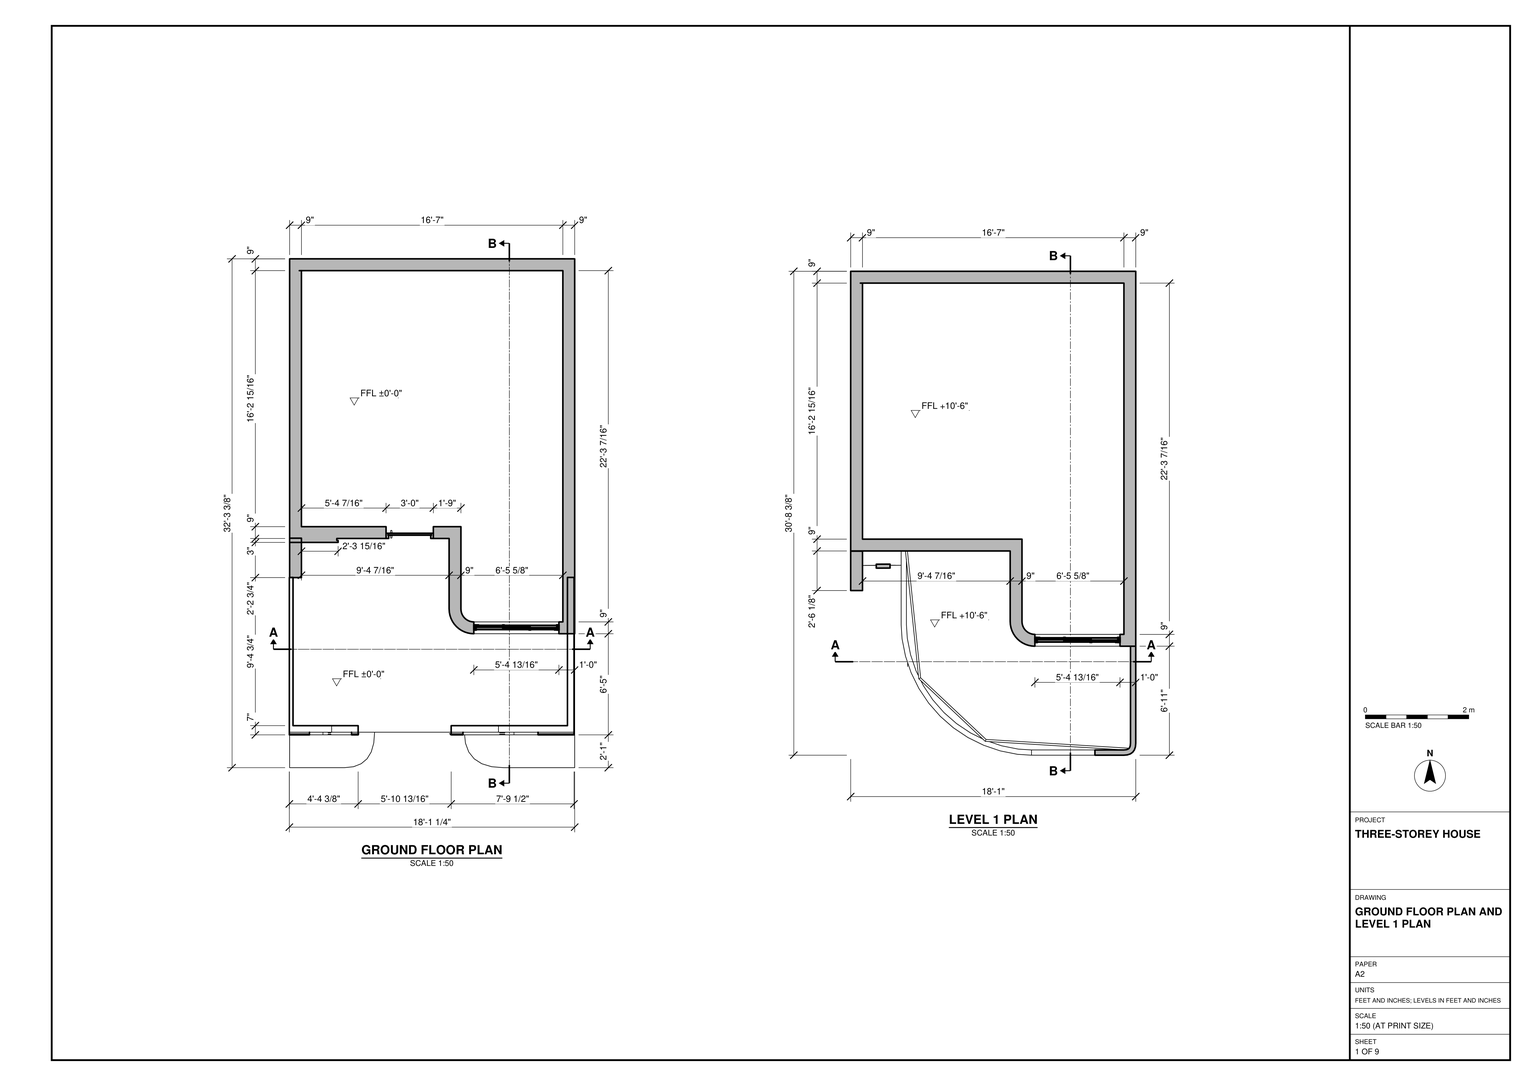
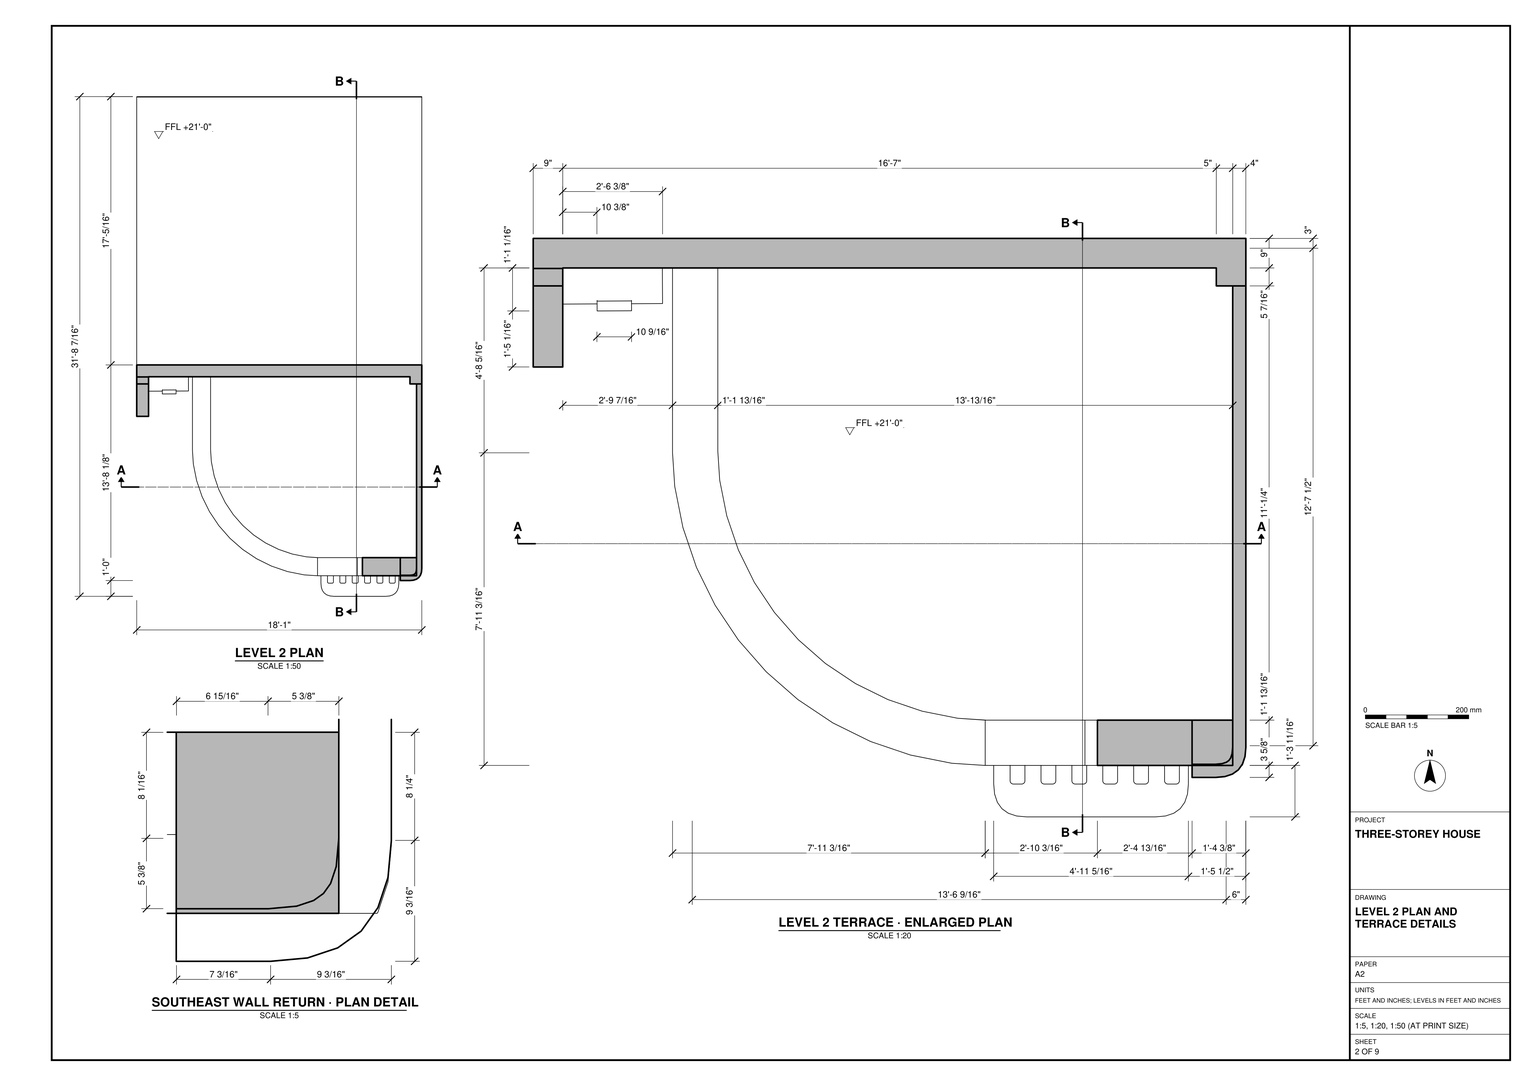
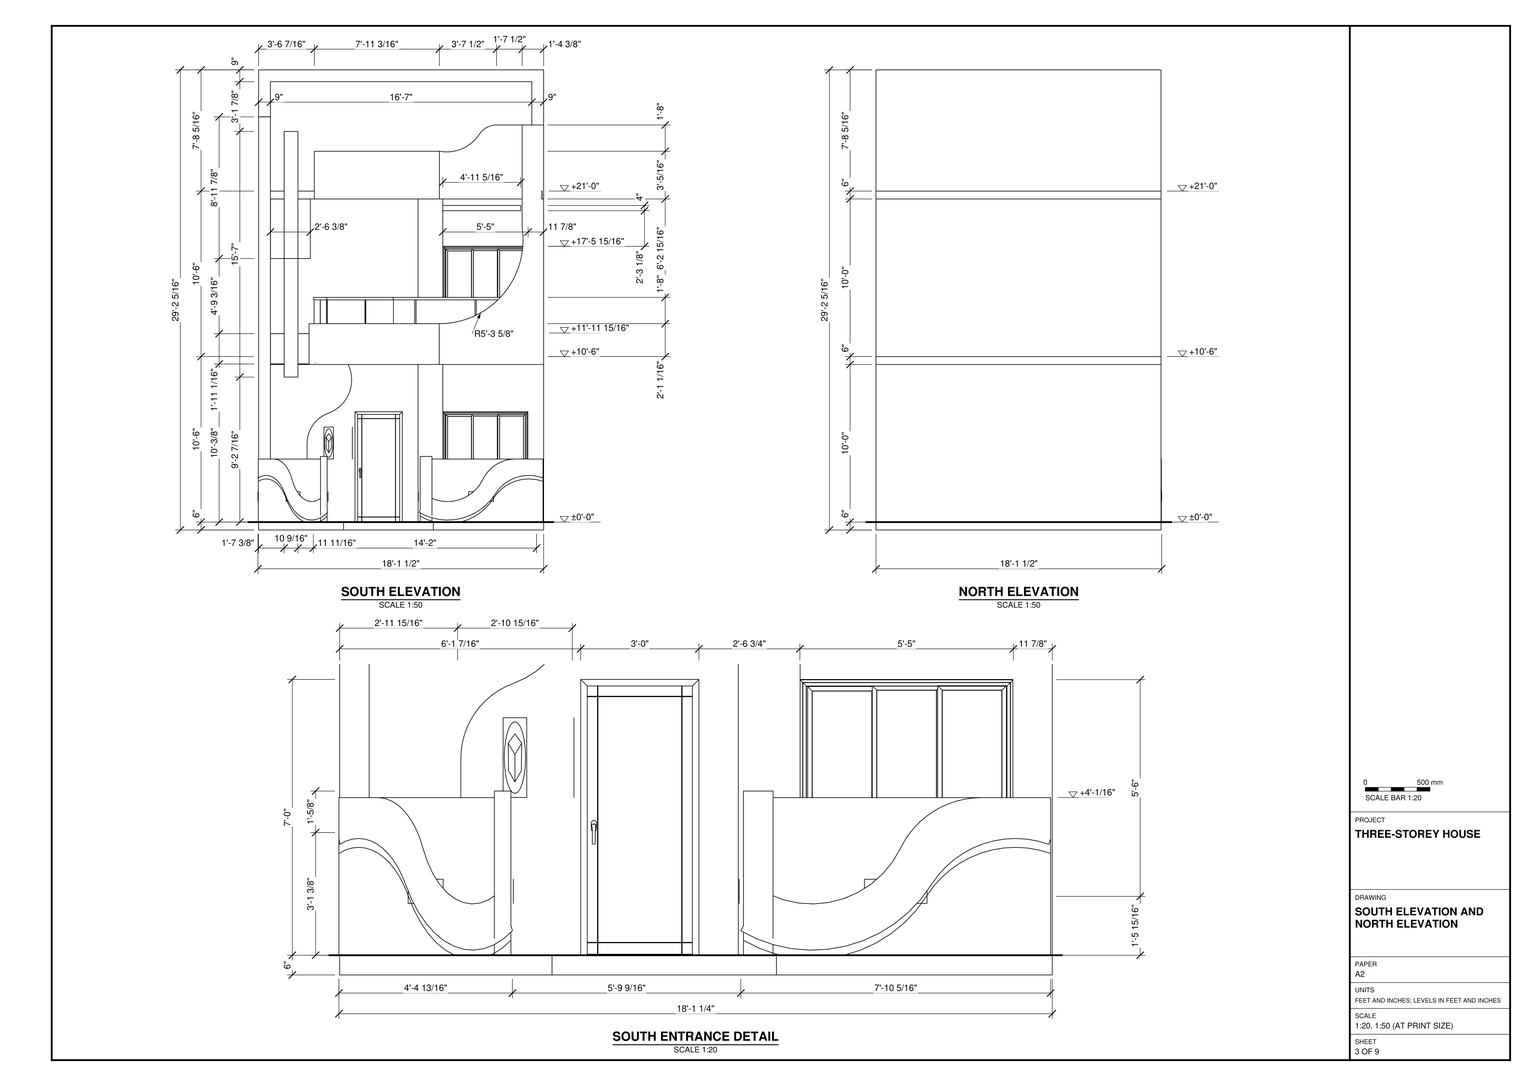
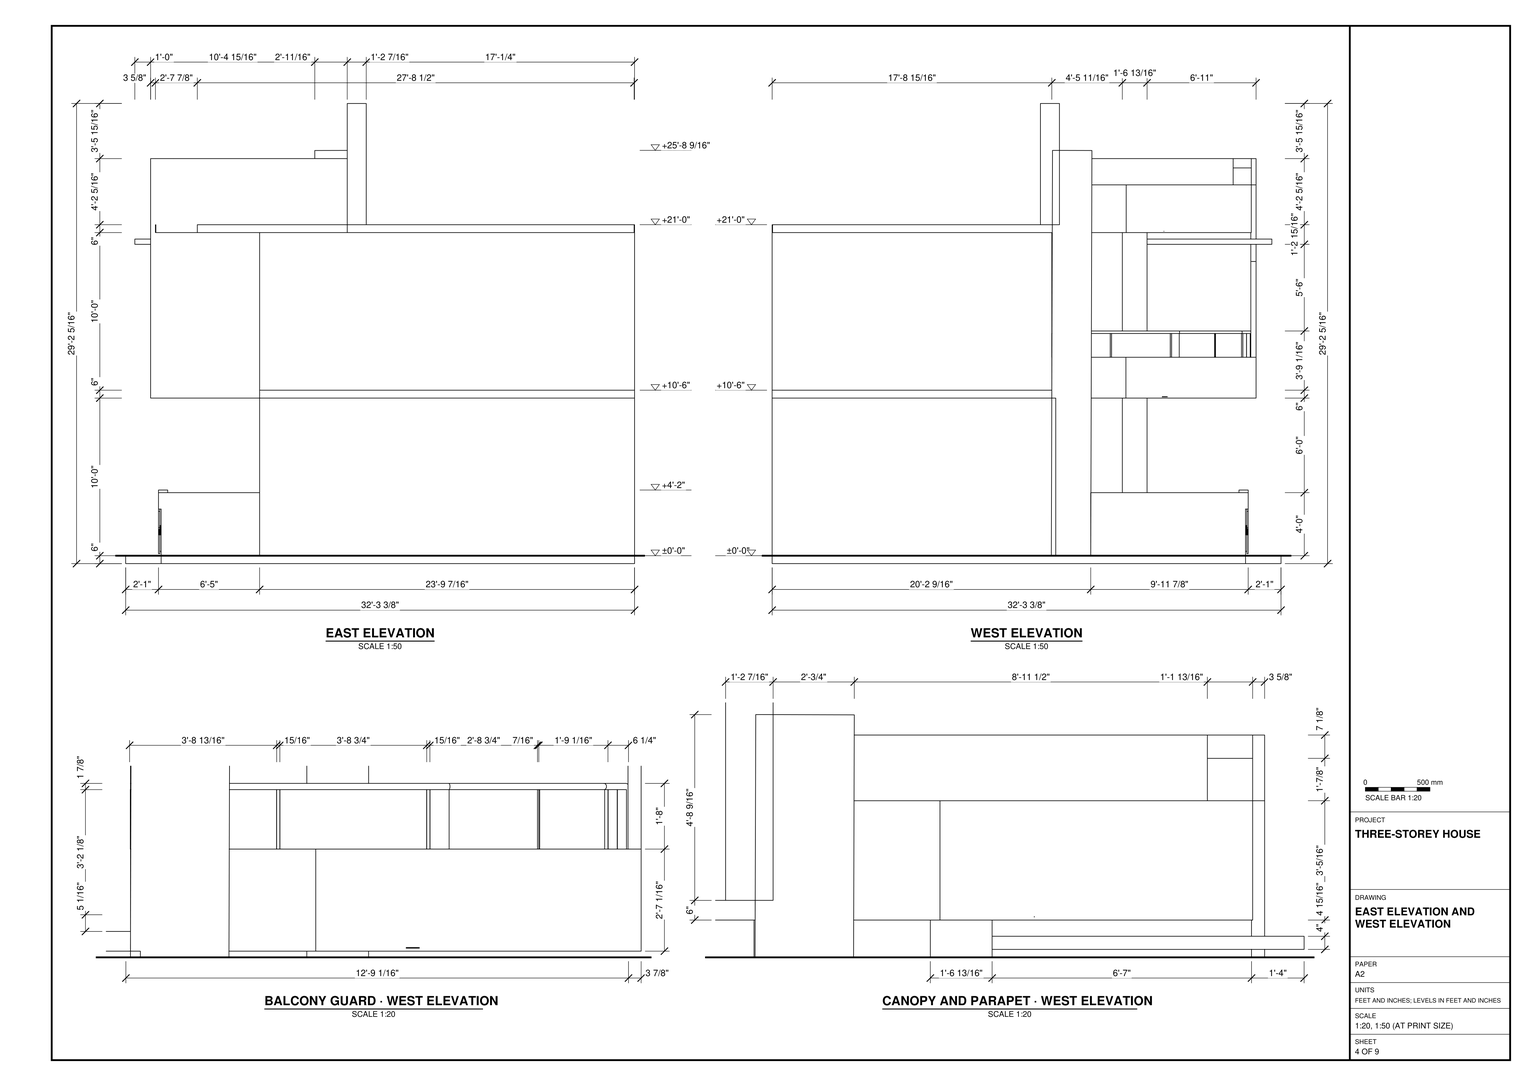
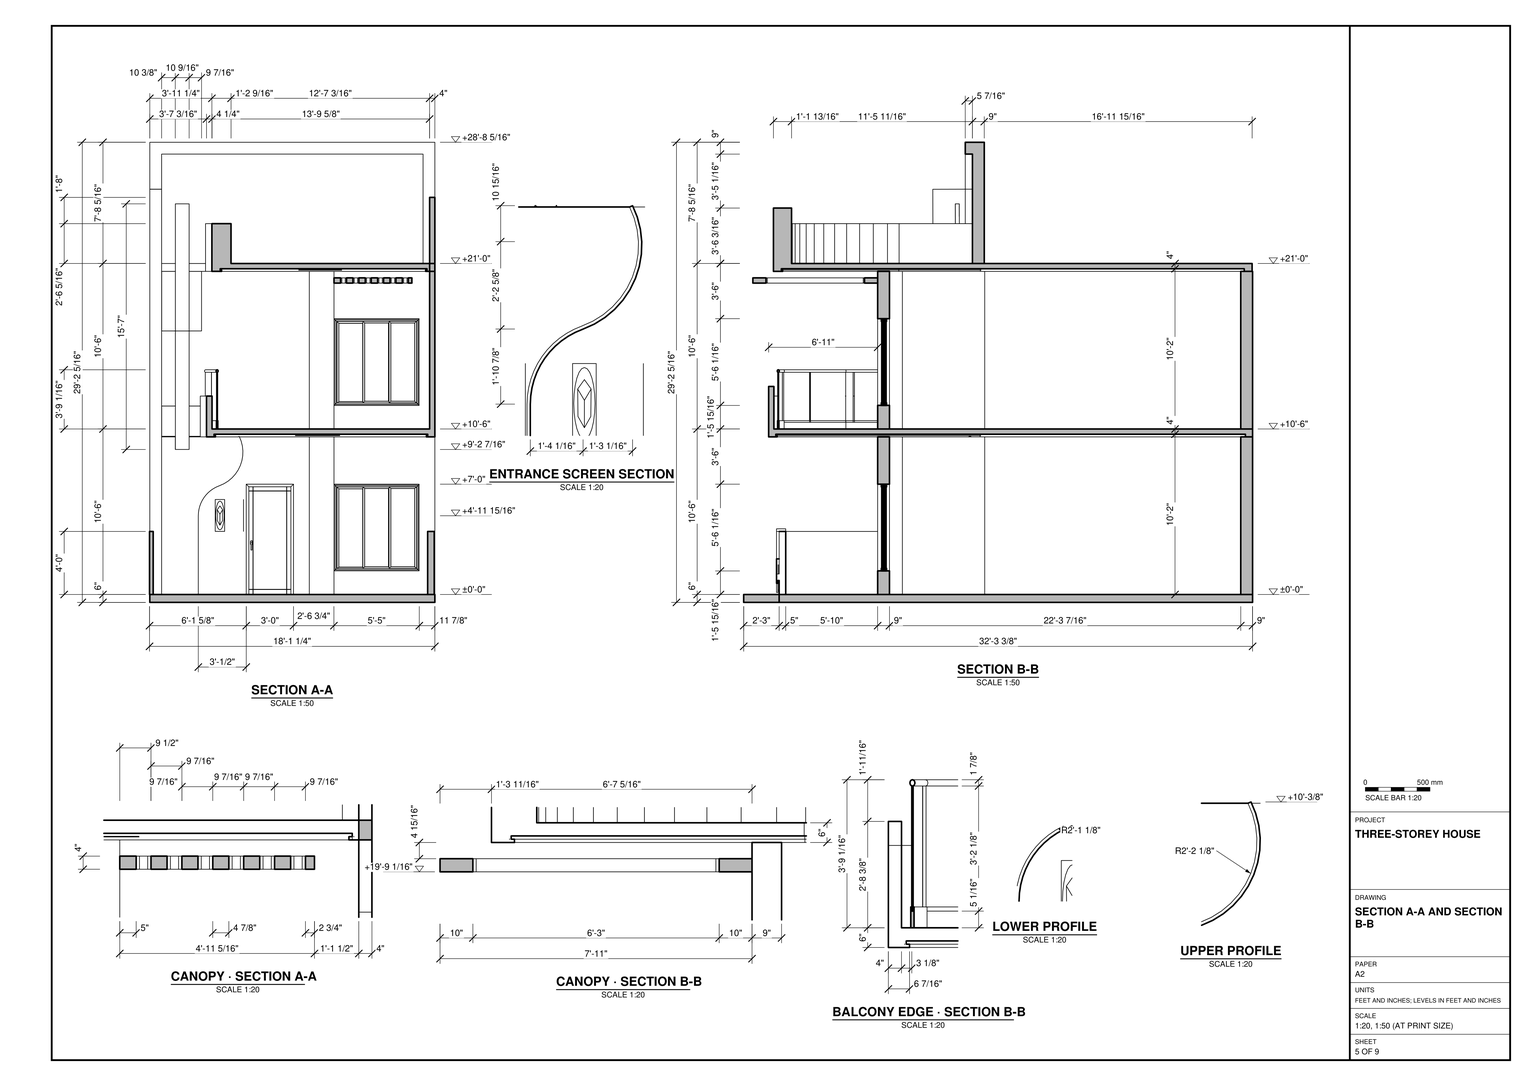
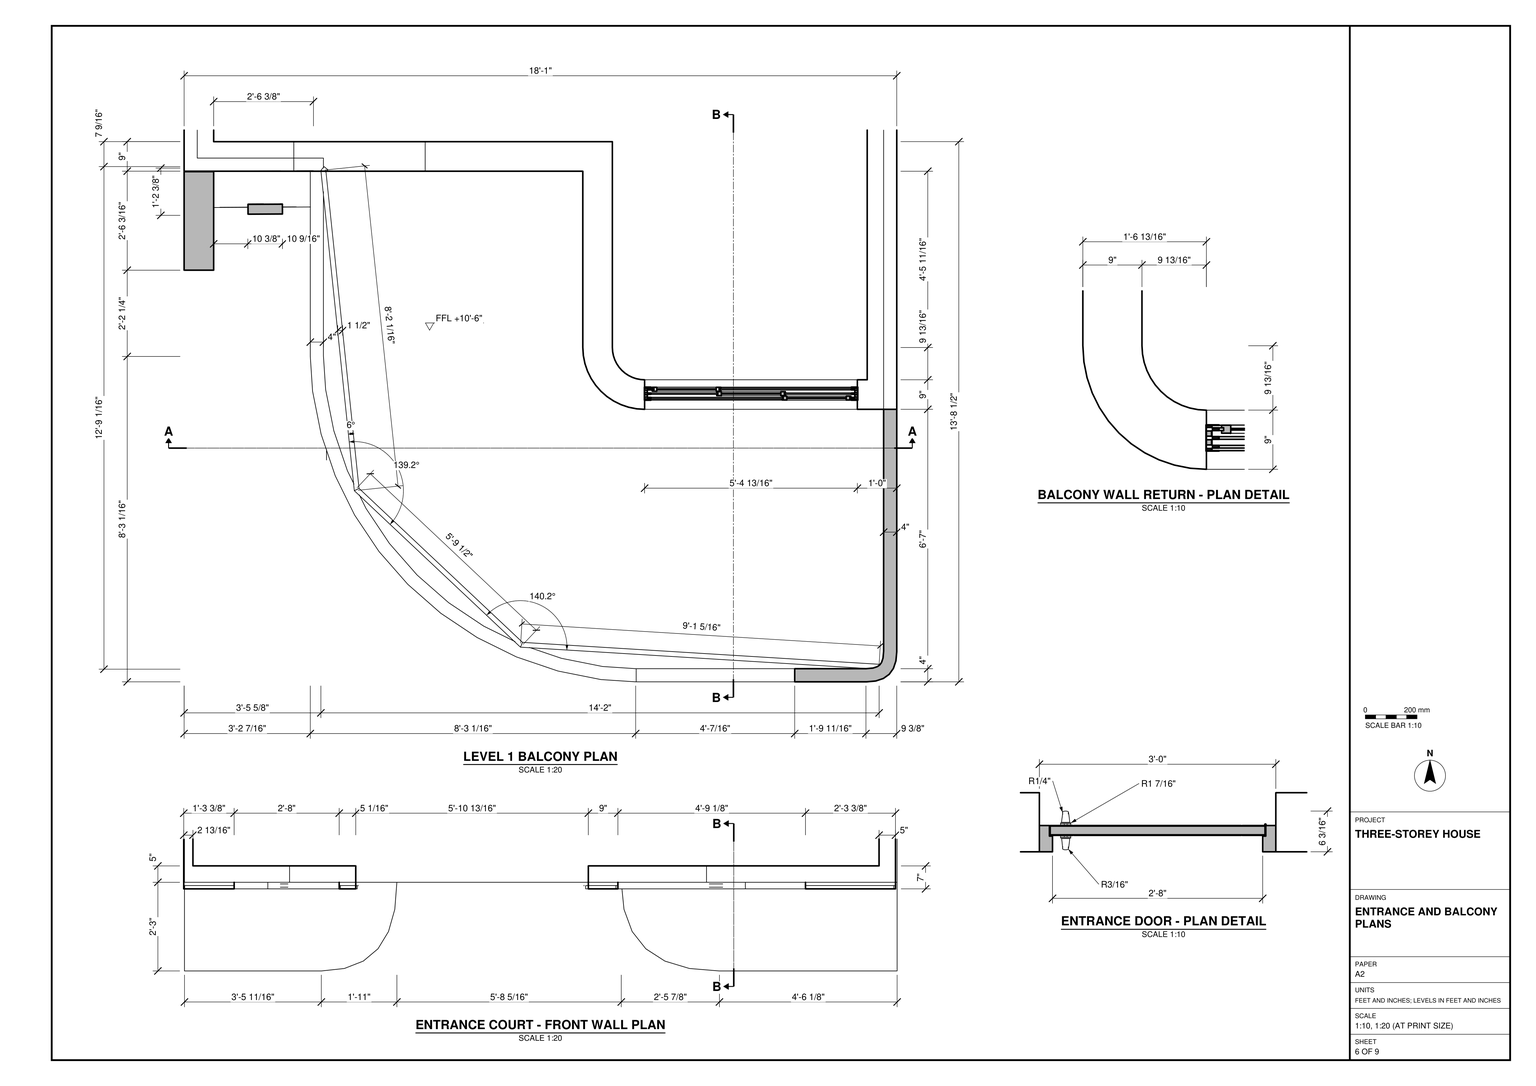
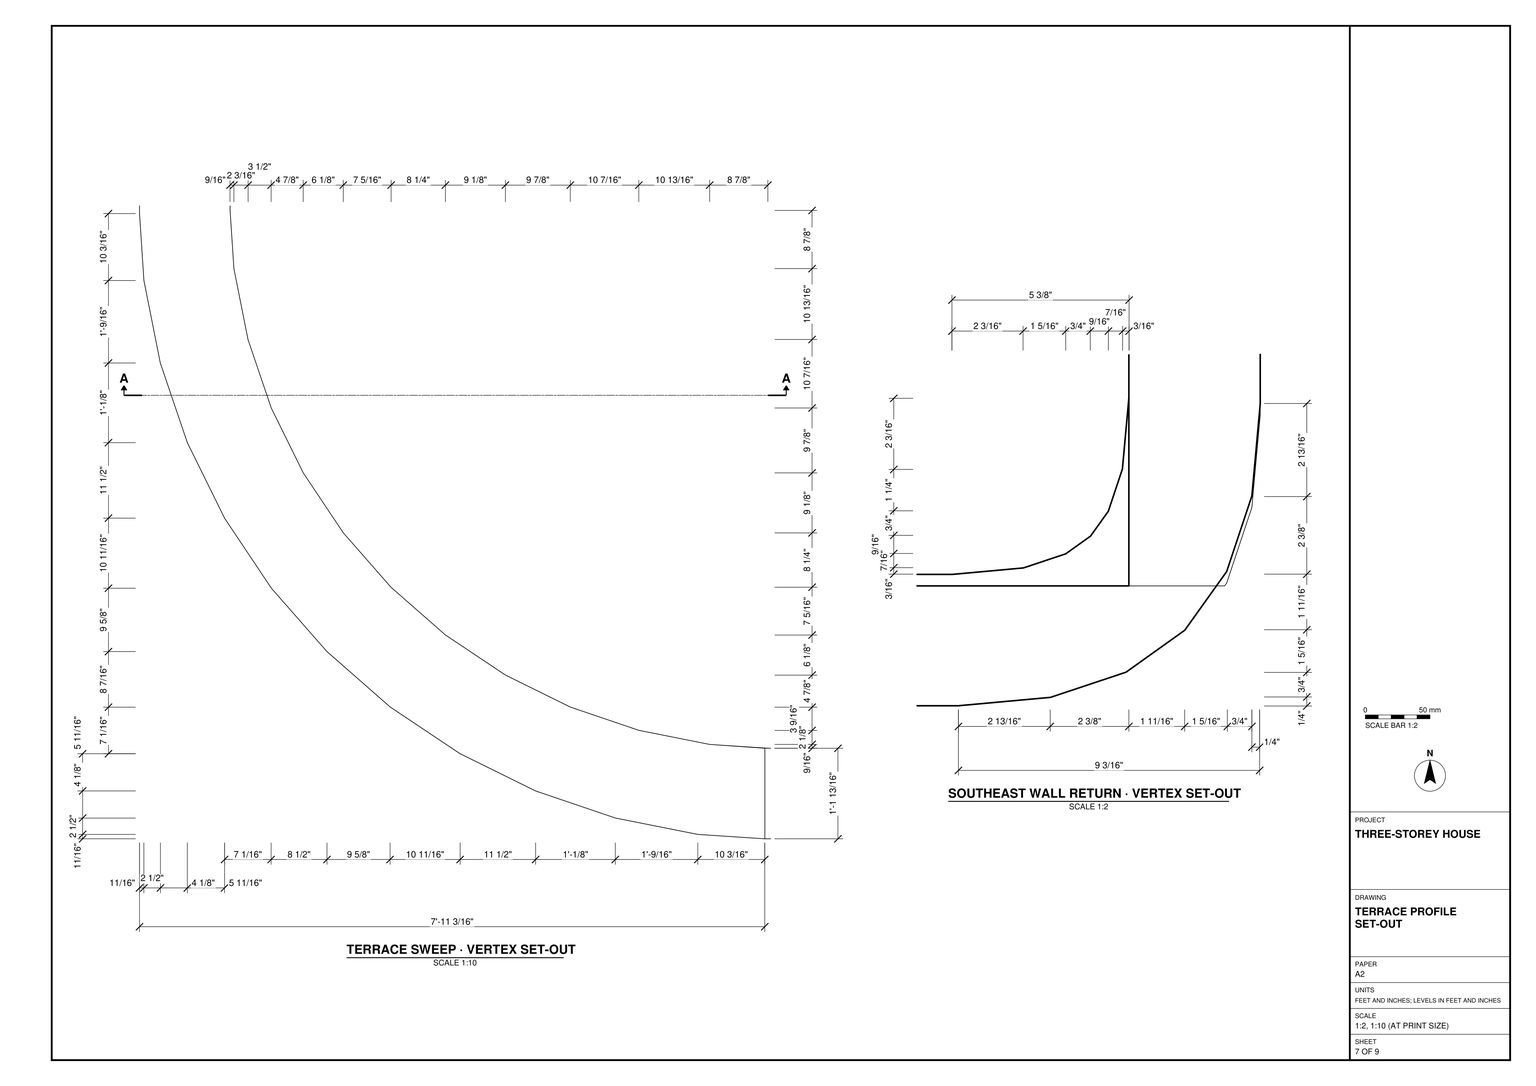
Build the three-storey house in SketchUp using task_files/diagram_01.pdf. Work in feet and inches. Set the overall east–west width to 18'-1 1/4", the north–south depth to 32'-3 3/8", and the height to 29'-2 5/16". Use finished floor levels of ±0'-0", +10'-6", and +21'-0".

Use the plans to lay out the rectangular rear volume and the stepped south wall. Give the walls their drawn thicknesses, including the 9" main walls, and model the floor slabs and flat roof with their edges visible as shown in elevation. Keep the north elevation free of openings. On the south side, set the entrance door back from the gap in the low front walls. Shape the sweeping profiles on either side of that gap and fit the framed window to the right of the door.

Use each upper-floor plan for its own terrace outline. Include the balcony railing, the tall narrow facade projection, and the rounded wall return at the southeast corner. Use separate groups or components for shell elements and for each furniture or joinery piece shown; use components for repeated parts. Decor and loose items shown may be any suitable library components. Save one SketchUp model as output_files/three_storey_house_with_curved_south_terraces.skp.

# SketchUp Ruby script. Lengths in inches.
U = 1.inch
M = Sketchup.active_model
def pt(a) = Geom::Point3d.new(a.map { |v| v * U })
def face(e, loops, mat)
  f = e.add_face(loops[0].map { |a| pt(a) })
  loops[1..].each { |l| e.add_face(l.map { |a| pt(a) }).erase! }
  f.material = f.back_material = mat if mat
  f
end
# faces: each face lists its corners as indices into pts; further lists are holes
def faces(e, pts, list, mat = nil) = list.each { |f| face(e, (f[0].is_a?(Array) ? f : [f]).map { |l| l.map { |i| pts[i] } }, mat) }
# xy, xz, yz: faces in a plane at the given z, y or x. An outline is a flat list of corners, or four numbers for a rectangle; further outlines are holes
def ring(l) = l.size == 4 ? [[l[0], l[1]], [l[2], l[1]], [l[2], l[3]], [l[0], l[3]]] : l.each_slice(2).to_a
def flat(e, list, mat, &to3) = list.each { |f| face(e, (f[0].is_a?(Array) ? f : [f]).map { |l| ring(l).map { |u, v| to3.(u, v) } }, mat) }
def xy(e, z, list, mat = nil) = flat(e, list, mat) { |x, y| [x, y, z] }
def xz(e, y, list, mat = nil) = flat(e, list, mat) { |x, z| [x, y, z] }
def yz(e, x, list, mat = nil) = flat(e, list, mat) { |y, z| [x, y, z] }
def lines(e, pts, list) = list.each { |a, b| e.add_line(pt(pts[a]), pt(pts[b])) }
# prism: a flat outline (further loops are holes) pulled along v
def prism(e, loops, v, mat = nil)
  f = face(e, loops, mat); d = Geom::Vector3d.new(v.map { |x| x * U })
  f.pushpull(f.normal.samedirection?(d) ? d.length : -d.length)
end
def box(e, o, s, mat = nil) = prism(e, [[o, [o[0] + s[0], o[1], o[2]], [o[0] + s[0], o[1] + s[1], o[2]], [o[0], o[1] + s[1], o[2]]]], [0, 0, s[2]], mat)
def at(x, y, z, deg = 0) = Geom::Transformation.translation(pt([x, y, z])) * Geom::Transformation.rotation(ORIGIN, Z_AXIS, deg.degrees)
def axes(o, x, y, z) = Geom::Transformation.new([*x, 0, *y, 0, *z, 0, *pt(o).to_a, 1])
def part(name) = M.definitions.add(name)
# library, detail: a bought-in or finely detailed component or shape, given as its bounding box
def library(name, o, s) = part(name).tap { |d| box(d.entities, o, s) }
def detail(e, o, s) = box(e.add_group.entities, o, s)
def put(e, d, t, mat = nil) = e.add_instance(d, t).tap { |i| i.material = mat if mat }
def group(e, t, mat = nil) = e.add_group.tap { |g| g.transformation = t; g.material = mat if mat }.entities
root = M.entities
M.materials.add("[Formica Graystone]").color = [149, 146, 135]
M.materials.add("[Formica Laminate Light]").color = [213, 189, 164]
M.materials.add("[Wood Cherry Original]").color = [152, 86, 42]
c1 = library("CTS_Window_Frame\#1",[1571.59,0.98,78.15],[65,4,66])
c2 = part("Group316\#3")
p = [[0,0,0],[0,0,-89.7],[-16.49,0,-89.7],[107.35,-183.05,0],[-107.35,-183.05,0],[107.35,183.05,0],
  [107.35,0,0],[-107.35,183.05,0],[16.49,0,-89.7],[-107.35,0,0],[0,0,-145.2]]
lines(c2.entities,p,[[0,1],[1,2],[3,4],[5,6],[7,5],[1,8],[9,0],[0,6],[8,10],[4,9],[6,3],[2,10],
  [9,7]])
c3 = part("Rectangle Light")
put(c3.entities,c2,at(0,0,0))
c4 = part("Group318\#1")
p = [[0,0,0],[0,0,-89.62],[-16.59,0,-89.62],[107.99,-182.15,0],[-107.99,-182.15,0],[107.99,182.15,0],
  [107.99,0,0],[-107.99,182.15,0],[16.59,0,-89.62],[-107.99,0,0],[0,0,-145.07]]
lines(c4.entities,p,[[0,1],[1,2],[3,4],[5,6],[7,5],[1,8],[9,0],[0,6],[8,10],[4,9],[6,3],[2,10],
  [9,7]])
c5 = part("Rectangle Light\#1")
put(c5.entities,c4,at(0,0,0))
c6 = library("Group123\#1",[-245.88,56.46,51.12],[36,6.2,84])
c7 = library("Group\#11",[-9.29,0,0],[59.29,4,95])
c8 = library("Group\#7",[-33.41,-82.98,0],[217.01,368.39,182.34])
c9 = library("Group\#10",[-0.5,-0.5,0],[35.9375,1,120.38])
c10 = library("Glass Railing\#2",[-169.4375,-0.78,0],[169.99,153.05,35.5])
c11 = library("Group297\#3",[-33.91,-76.98,0],[95.34,119.86,50])
c12 = library("Group297\#2",[-33.91,-76.98,0],[95.34,119.86,50])
c13 = library("Group\#9",[-0.5,-0.5,-0.1],[163.58,152.49,0.2])
c14 = part("Group\#13")
prism(c14.entities,[[[0,0,0],[0,27,0],[84,27,0],[83.17,18.75,0],[80.68,12,0],[76.53,6.75,0],[70.71,3,0],[63.24,0.75,0],[54.1,0,0]]],[0,0,6])
xy(root,48,[[132.2,27,195.57,32]])
xy(root,252,[[213.23,54.54,217.23,59.29]])
xz(root,32,[[123.2,0,211.73,48]])
xz(root,36.44,[[137.85,252,137.85,282.34,138.31,282.28,138.31,252]])
xz(root,54.54,[[213.23,246,217.23,252]])
yz(root,217.23,[[54.54,246,387.4,252]])
# 12 loose lines left out
p = [[129.46,37.02,252],[129.46,37.02,282.34],[137.85,36.44,282.34],[137.85,36.44,252]]
faces(root,p,[[0,1,2,3]])
put(root,c1,at(-1431.22,103.77,-60.22))
put(root,c1,at(-1431.22,103.77,65.78))
put(root,c3,axes([107.57,204.35,119.99],[1,0,0],[0,-1,0],[0,0,1]))
put(root,c5,axes([108.21,204.89,245.99],[1,0,0],[0,-1,0],[0,0,1]))
put(root,c6,axes([-136.25,118.03,-51.12],[-1,0,0],[0,1,0],[0,0,1]),"[Wood Cherry Original]")
g1 = group(root,at(33.625,101.98,126))
xy(g1,0,[[106.8125,0,104.36,0.16,101.94,0.64,99.61,1.43,97.41,2.52,95.36,3.89,93.51,5.51,91.89,7.36,90.52,9.41,89.43,11.61,88.64,13.94,88.16,16.36,88,18.8125,88,72.51,40,72.51,40,81.51,97,81.51,97,18.8125,97.08,17.53,97.33,16.27,97.75,15.06,98.31,13.91,99.03,12.84,99.875,11.875,100.84,11.03,101.91,10.31,103.06,9.75,104.27,9.33,105.53,9.08,106.8125,9,174.6,9,174.6,276.41,0,276.41,0,285.41,183.6,285.41,183.6,0],[-33.41,72.51,-33.41,285.41,0,285.41,0,276.41,-24.41,276.41,-24.41,81.51,0,81.51,0,72.51],[0,72.51,40,81.51]])
xy(g1,18,[[106.8125,0,171.6,9]])
xy(g1,84,[[106.8125,0,171.6,9]])
xy(g1,120,[[[106.8125,0,183.6,0,183.6,285.41,-33.41,285.41,-33.41,72.51,88,72.51,88,18.8125,88.16,16.36,88.64,13.94,89.43,11.61,90.52,9.41,91.89,7.36,93.51,5.51,95.36,3.89,97.41,2.52,99.61,1.43,101.94,0.64,104.36,0.16],[106.8125,9,105.53,9.08,104.27,9.33,103.06,9.75,101.91,10.31,100.84,11.03,99.875,11.875,99.03,12.84,98.31,13.91,97.75,15.06,97.33,16.27,97.08,17.53,97,18.8125,97,81.51,-24.41,81.51,-24.41,276.41,174.6,276.41,174.6,9]]])
xz(g1,0,[[106.8125,0,183.6,0,183.6,120,106.8125,120,106.8125,84,171.6,84,171.6,18,106.8125,18]])
xz(g1,9,[[106.8125,0,106.8125,18,171.6,18,171.6,84,106.8125,84,106.8125,120,174.6,120,174.6,0]])
xz(g1,72.51,[[-33.41,0,88,120]])
xz(g1,81.51,[[-24.41,0,97,120]])
xz(g1,276.41,[[-26.08,0,-24.41,120],[-24.41,0,174.6,120]])
xz(g1,285.41,[[-33.41,0,183.6,120]])
yz(g1,-33.41,[[42.875,-126.09,41.97,182.5,71.97,182.58,72.51,0,72.875,-126],[72.51,0,285.41,120]])
yz(g1,-24.41,[[42.875,-126.09,72.875,-126,72.51,0,71.97,182.58,41.97,182.5],[81.51,0,276.41,120]])
yz(g1,88,[[18.8125,0,72.51,120]])
yz(g1,97,[[18.8125,0,81.51,120]])
yz(g1,106.8125,[[0,18,9,84]])
yz(g1,171.6,[[0,18,9,84]])
yz(g1,174.6,[[9,0,276.41,120]])
yz(g1,183.6,[[0,0,285.41,120]])
p = [[-24.41,41.97,182.5],[-33.41,41.97,182.5],[-33.41,42.875,-126.09],[-24.41,42.875,-126.09],[-33.41,72.875,-126],[-24.41,72.875,-126],
  [-33.41,72.51,0],[-24.41,72.51,0],[104.36,0.16,0],[106.8125,0,0],[106.8125,0,18],[106.8125,0,84],
  [106.8125,0,120],[104.36,0.16,120],[101.94,0.64,0],[101.94,0.64,120],[99.61,1.43,0],[99.61,1.43,120],
  [97.41,2.52,0],[97.41,2.52,120],[95.36,3.89,0],[95.36,3.89,120],[93.51,5.51,0],[93.51,5.51,120],
  [91.89,7.36,0],[91.89,7.36,120],[90.52,9.41,0],[90.52,9.41,120],[106.8125,9,0],[105.53,9.08,0],
  [105.53,9.08,120],[106.8125,9,120],[106.8125,9,84],[106.8125,9,18],[104.27,9.33,0],[104.27,9.33,120],
  [103.06,9.75,0],[103.06,9.75,120],[89.43,11.61,0],[89.43,11.61,120],[101.91,10.31,0],[101.91,10.31,120],
  [100.84,11.03,0],[100.84,11.03,120],[99.875,11.875,0],[99.875,11.875,120],[88.64,13.94,0],[88.64,13.94,120],
  [99.03,12.84,0],[99.03,12.84,120],[98.31,13.91,0],[98.31,13.91,120],[88.16,16.36,0],[88.16,16.36,120],
  [97.75,15.06,0],[97.75,15.06,120],[97.33,16.27,0],[97.33,16.27,120],[97.08,17.53,0],[97.08,17.53,120],
  [88,18.8125,0],[88,18.8125,120],[97,18.8125,0],[97,18.8125,120],[-33.41,71.97,182.58],[-24.41,71.97,182.58]]
faces(g1,p,[[0,1,2,3],[4,5,3,2],[6,7,5,4],[8,9,10,11,12,13],[14,8,13,15],[16,14,15,17],[18,16,17,19],[20,18,19,21],
  [22,20,21,23],[24,22,23,25],[26,24,25,27],[28,29,30,31,32,33],[29,34,35,30],[34,36,37,35],[38,26,27,39],[36,40,41,37],
  [40,42,43,41],[42,44,45,43],[46,38,39,47],[44,48,49,45],[48,50,51,49],[52,46,47,53],[50,54,55,51],[54,56,57,55],
  [56,58,59,57],[60,52,53,61],[58,62,63,59],[64,65,7,6],[1,0,65,64]])
g2 = group(g1,at(-24.41,72.34,57.67),"[Formica Graystone]")
prism(g2,[[[0,0.18,-63.22],[30.33,0.35,-63.22],[30.39,-10.65,-63.25],[0.0625,-10.81,-63.25]]],[0,-0.07,23.04])
# 1 loose lines left out
p = [[0.0625,-11.18,62.3],[-0.01,0.82,62.33],[-0.01,0.95,17.01],[0,-0.05,17],[0.0625,-11.05,16.97],[10.46,-10.99,16.97],
  [10.46,-11.125,62.3],[30.39,-11.01,62.3],[20.9375,-11.07,62.3],[20.9375,-10.93,16.97],[30.39,-10.88,16.97],[30.32,1.12,17.01],
  [30.32,0.99,62.33]]
faces(g2,p,[[0,1,2,3,4],[4,5,6,0],[7,8,9,10],[10,9,5,4,3,2,11],[10,11,12,7],[12,11,2,1],[7,12,1,0,6,8]])
g3 = group(g2,at(10.46,-10.93,16.97),"[Formica Laminate Light]")
p = [[-0.01,0.94,0],[-0.01,1.18,-80.22],[-0.06,11.03,-80.1875],[-0.06,11.0625,-90.1875],[0.01,-1.79,-90.23],[0.01,-2.06,-0.01],
  [10.49,-1.74,-90.23],[10.49,-2,-0.01],[10.42,11.12,-90.1875],[10.42,11.09,-80.1875],[10.48,1.23,-80.22],[10.48,1,0],
  [10.49,-2.28,96.77],[0.01,-2.34,96.77],[-0.01,0.66,96.78],[10.48,0.72,96.78]]
faces(g3,p,[[0,1,2,3,4,5],[5,4,6,7],[7,6,8,9,10,11],[8,6,4,3],[3,2,9,8],[11,10,1,0],[1,10,9,2],[12,13,5,7],
  [13,14,0,5],[15,12,7,11],[5,7,11,0],[14,15,11,0],[14,13,12,15]])
put(g1,c7,axes([116.1,0,111.06],[1,0,0],[0,0,1],[0,-1,0]))
put(root,c8,at(33.625,101.98,120))
g4 = group(root,at(29.625,105.98,-6))
xy(g4,0,[[-29.41,-78.98,-29.41,281.41,187.6,281.41,187.6,-78.98,178.93,-78.98,178.93,-75.77,174.22,-75.77,174.22,-78.98],[174.22,-78.98,174.22,-75.77,178.93,-75.77,178.93,-77.125,178.43,-77.82,177.68,-78.36,176.39,-78.79],[174.22,-78.98,176.39,-78.79,177.68,-78.36,178.43,-77.82,178.93,-77.125,178.93,-78.98]])
xy(g4,6,[[-29.41,-78.98,187.6,281.41]])
xz(g4,-78.98,[[-29.41,0,187.6,6]])
xz(g4,281.41,[[-29.41,0,187.6,6]])
yz(g4,-29.41,[[-78.98,0,281.41,6]])
yz(g4,187.6,[[-78.98,0,281.41,6]])
g5 = group(root,at(33.625,101.98,0))
xy(g5,0,[[106.8125,0,104.36,0.16,101.94,0.64,99.61,1.43,97.41,2.52,95.36,3.89,93.51,5.51,91.89,7.36,90.52,9.41,89.43,11.61,88.64,13.94,88.16,16.36,88,18.8125,88,72.51,76,72.51,76,81.51,97,81.51,97,18.8125,97.08,17.53,97.33,16.27,97.75,15.06,98.31,13.91,99.03,12.84,99.875,11.875,100.84,11.03,101.91,10.31,103.06,9.75,104.27,9.33,105.53,9.08,106.8125,9,174.6,9,174.6,276.41,0,276.41,0,285.41,183.6,285.41,183.6,0],[-33.41,69.51,-33.41,285.41,0,285.41,0,276.41,-24.41,276.41,-24.41,81.51,0,81.51,0,69.51],[0,69.51,0,81.51,40,81.51,40,72.51,2.51,72.51,2.51,69.51],[2.51,69.51,3.51,71.01]])
xy(g5,18,[[106.8125,0,171.6,9]])
xy(g5,84,[[106.8125,0,171.6,9],[40,72.51,76,81.51]])
xy(g5,120,[[[106.8125,0,183.6,0,183.6,285.41,-33.41,285.41,-33.41,69.51,33.73,69.51,33.73,72.51,88,72.51,88,18.8125,88.16,16.36,88.64,13.94,89.43,11.61,90.52,9.41,91.89,7.36,93.51,5.51,95.36,3.89,97.41,2.52,99.61,1.43,101.94,0.64,104.36,0.16],[106.8125,9,105.53,9.08,104.27,9.33,103.06,9.75,101.91,10.31,100.84,11.03,99.875,11.875,99.03,12.84,98.31,13.91,97.75,15.06,97.33,16.27,97.08,17.53,97,18.8125,97,81.51,-24.41,81.51,-24.41,276.41,174.6,276.41,174.6,9]]])
xz(g5,0,[[106.8125,0,183.6,0,183.6,120,106.8125,120,106.8125,84,171.6,84,171.6,18,106.8125,18]])
xz(g5,9,[[106.8125,0,106.8125,18,171.6,18,171.6,84,106.8125,84,106.8125,120,174.6,120,174.6,0]])
xz(g5,69.51,[[-33.41,0,3.51,0,3.51,59.97,3.64,62.47,4.01,64.91,4.64,67.3,5.5,69.62,6.6,71.83,7.91,73.92,9.43,75.87,11.14,77.65,13.03,79.25,15.07,80.65,17.24,81.83,19.57,82.81,23,84.33,26.24,86.35,29.16,88.8,31.72,91.63,33.84,94.8,35.51,98.23,36.68,101.86,37.33,105.62,37.44,109.43,37.03,113.22,36.08,116.92,34.66,120.38,33.73,120,-33.41,120]])
xz(g5,72.51,[[2.51,0,40,0,40,84,76,84,76,0,88,0,88,120,33.73,120,35.13,116.6,36.04,113.04,36.44,109.39,36.33,105.72,35.71,102.1,34.58,98.6,32.98,95.3,30.92,92.25,28.47,89.52,25.65,87.16,22.53,85.22,19.17,83.73,16.8,82.74,14.54,81.5,12.42,80.05,10.46,78.38,8.68,76.53,7.09,74.5,5.72,72.32,4.58,70.01,3.68,67.6,3.03,65.11,2.64,62.57,2.51,60]])
xz(g5,81.51,[[-24.41,0,-24.41,120,97,120,97,0,76,0,76,84,40,84,40,0]])
xz(g5,276.41,[[-26.08,0,-24.41,120],[-24.41,0,174.6,120]])
xz(g5,285.41,[[-33.41,0,183.6,120]])
yz(g5,-33.41,[[69.51,0,285.41,120]])
yz(g5,-24.41,[[81.51,0,276.41,120]])
yz(g5,2.51,[[71.01,0,72.51,60]])
yz(g5,3.51,[[69.51,0,71.01,59.97]])
yz(g5,40,[[72.51,0,81.51,84]])
yz(g5,76,[[72.51,0,81.51,84]])
yz(g5,88,[[18.8125,0,72.51,120]])
yz(g5,97,[[18.8125,0,81.51,120]])
yz(g5,106.8125,[[0,18,9,84]])
yz(g5,171.6,[[0,18,9,84]])
yz(g5,174.6,[[9,0,276.41,120]])
yz(g5,183.6,[[0,0,285.41,120]])
# 2 loose lines left out
p = [[104.36,0.16,0],[106.8125,0,0],[106.8125,0,18],[106.8125,0,84],[106.8125,0,120],[104.36,0.16,120],
  [101.94,0.64,0],[101.94,0.64,120],[99.61,1.43,0],[99.61,1.43,120],[97.41,2.52,0],[97.41,2.52,120],
  [95.36,3.89,0],[95.36,3.89,120],[93.51,5.51,0],[93.51,5.51,120],[91.89,7.36,0],[91.89,7.36,120],
  [90.52,9.41,0],[90.52,9.41,120],[106.8125,9,0],[105.53,9.08,0],[105.53,9.08,120],[106.8125,9,120],
  [106.8125,9,84],[106.8125,9,18],[104.27,9.33,0],[104.27,9.33,120],[103.06,9.75,0],[103.06,9.75,120],
  [89.43,11.61,0],[89.43,11.61,120],[101.91,10.31,0],[101.91,10.31,120],[100.84,11.03,0],[100.84,11.03,120],
  [99.875,11.875,0],[99.875,11.875,120],[88.64,13.94,0],[88.64,13.94,120],[99.03,12.84,0],[99.03,12.84,120],
  [98.31,13.91,0],[98.31,13.91,120],[88.16,16.36,0],[88.16,16.36,120],[97.75,15.06,0],[97.75,15.06,120],
  [97.33,16.27,0],[97.33,16.27,120],[97.08,17.53,0],[97.08,17.53,120],[88,18.8125,0],[88,18.8125,120],
  [97,18.8125,0],[97,18.8125,120],[3.51,69.51,59.97],[3.51,71.01,59.97],[3.64,71.01,62.47],[3.64,69.51,62.47],
  [2.64,72.51,62.57],[2.64,71.01,62.57],[2.51,71.01,60],[2.51,72.51,60],[4.01,71.01,64.91],[4.01,69.51,64.91],
  [3.03,72.51,65.11],[3.03,71.01,65.11],[4.64,71.01,67.3],[4.64,69.51,67.3],[3.68,72.51,67.6],[3.68,71.01,67.6],
  [5.5,71.01,69.62],[5.5,69.51,69.62],[4.58,72.51,70.01],[4.58,71.01,70.01],[6.6,71.01,71.83],[6.6,69.51,71.83],
  [5.72,72.51,72.32],[5.72,71.01,72.32],[7.91,71.01,73.92],[7.91,69.51,73.92],[7.09,72.51,74.5],[7.09,71.01,74.5],
  [9.43,71.01,75.87],[9.43,69.51,75.87],[8.68,72.51,76.53],[8.68,71.01,76.53],[11.14,69.51,77.65],[11.14,71.01,77.65],
  [10.46,72.51,78.38],[10.46,71.01,78.38],[13.03,71.01,79.25],[13.03,69.51,79.25],[12.42,72.51,80.05],[12.42,71.01,80.05],
  [15.07,71.01,80.65],[15.07,69.51,80.65],[14.54,72.51,81.5],[14.54,71.01,81.5],[17.24,71.01,81.83],[17.24,69.51,81.83],
  [16.8,72.51,82.74],[16.8,71.01,82.74],[19.57,71.01,82.81],[19.57,69.51,82.81],[19.17,72.51,83.73],[19.17,71.01,83.73],
  [23,71.01,84.33],[23,69.51,84.33],[22.53,72.51,85.22],[22.53,71.01,85.22],[26.24,71.01,86.35],[26.24,69.51,86.35],
  [25.65,72.51,87.16],[25.65,71.01,87.16],[29.16,71.01,88.8],[29.16,69.51,88.8],[28.47,72.51,89.52],[28.47,71.01,89.52],
  [31.72,69.51,91.63],[31.72,71.01,91.63],[30.92,72.51,92.25],[30.92,71.01,92.25],[33.84,69.51,94.8],[33.84,71.01,94.8],
  [32.98,72.51,95.3],[32.98,71.01,95.3],[35.51,71.01,98.23],[35.51,69.51,98.23],[34.58,72.51,98.6],[34.58,71.01,98.6],
  [36.68,71.01,101.86],[36.68,69.51,101.86],[35.71,72.51,102.1],[35.71,71.01,102.1],[37.33,71.01,105.62],[37.33,69.51,105.62],
  [36.33,72.51,105.72],[36.33,71.01,105.72],[37.44,71.01,109.43],[37.44,69.51,109.43],[36.44,72.51,109.39],[36.44,71.01,109.39],
  [37.03,71.01,113.22],[37.03,69.51,113.22],[36.04,72.51,113.04],[36.04,71.01,113.04],[35.13,72.51,116.6],[35.13,71.01,116.6],
  [36.08,71.01,116.92],[36.08,69.51,116.92],[33.73,72.51,120],[33.73,71.01,120],[34.66,71.01,120.38],[34.66,69.51,120.38],
  [33.73,69.51,120]]
faces(g5,p,[[0,1,2,3,4,5],[6,0,5,7],[8,6,7,9],[10,8,9,11],[12,10,11,13],[14,12,13,15],[16,14,15,17],[18,16,17,19],
  [20,21,22,23,24,25],[21,26,27,22],[26,28,29,27],[30,18,19,31],[28,32,33,29],[32,34,35,33],[34,36,37,35],[38,30,31,39],
  [36,40,41,37],[40,42,43,41],[44,38,39,45],[42,46,47,43],[46,48,49,47],[48,50,51,49],[52,44,45,53],[50,54,55,51],
  [56,57,58,59],[60,61,62,63],[59,58,64,65],[66,67,61,60],[65,64,68,69],[70,71,67,66],[69,68,72,73],[74,75,71,70],
  [73,72,76,77],[78,79,75,74],[77,76,80,81],[82,83,79,78],[81,80,84,85],[86,87,83,82],[88,85,84,89],[90,91,87,86],
  [88,89,92,93],[94,95,91,90],[93,92,96,97],[98,99,95,94],[97,96,100,101],[102,103,99,98],[101,100,104,105],[106,107,103,102],
  [105,104,108,109],[110,111,107,106],[109,108,112,113],[114,115,111,110],[113,112,116,117],[118,119,115,114],[120,117,116,121],[122,123,119,118],
  [124,120,121,125],[126,127,123,122],[124,125,128,129],[130,131,127,126],[129,128,132,133],[134,135,131,130],[133,132,136,137],[138,139,135,134],
  [137,136,140,141],[142,143,139,138],[141,140,144,145],[146,147,143,142],[148,149,147,146],[145,144,150,151],[152,153,149,148],[151,150,154,155],
  [156,155,154,153]])
put(g5,c9,at(2.51,71.01,0))
put(root,c10,axes([211.3,23.625,126],[1,0,0],[0,1,0],[0,0,1.27]))
put(root,c11,axes([18.71,101.98,0],[0.56,0,0],[0,1,0],[0,0,1]))
put(root,c12,axes([183.32,101.98,0],[-1,0,0],[0,1,0],[0,0,1]))
g6 = group(root,at(0.22,101.63,246))
xy(g6,0,[[[137.63,-78.98,127.43,-78.31,114.86,-75.81,102.73,-71.7,91.24,-66.03,80.58,-58.91,70.95,-50.46,62.5,-40.82,55.38,-30.17,49.71,-18.68,45.59,-6.54,43.09,6.03,42.42,16.23,42.42,72.51,0,72.51,0,285.41,217.01,285.41,217.01,-73.79,216.75,-76.6,215.98,-78.9,215.92,-78.98],[137.86,-71.98,210.01,-71.98,210.01,0.21,211.01,0.21,211.01,279.41,6,279.41,6,78.51,49.42,78.51,49.42,16.46,50.05,6.94,52.37,-4.73,56.19,-15.99,61.45,-26.66,68.0625,-36.55,75.91,-45.5,84.85,-53.34,94.74,-59.95,105.41,-65.21,116.68,-69.04,128.35,-71.36]]])
xy(g6,2,[[137.83,-72.98,128.22,-72.35,116.42,-70.01,105.03,-66.14,94.24,-60.82,84.24,-54.14,75.2,-46.21,67.27,-37.16,60.59,-27.16,55.27,-16.375,51.4,-4.99,49.05,6.8125,48.42,16.43,48.42,78.51,6,78.51,6,279.41,211.01,279.41,211.01,-72.98]])
xy(g6,6,[[200.63,-78.98,213.01,-65.19],[138.09,-65.19,213.01,-65.19,213.01,-42.69,217.01,-42.69,217.01,67.04,208.01,67.04,208.01,72.51,56.21,72.51,56.21,16.68,56.79,7.83,58.94,-2.96,62.48,-13.39,67.35,-23.26,73.46,-32.41,80.72,-40.6875,89,-47.94,98.15,-54.06,108.02,-58.93,118.44,-62.46,129.24,-64.61],[0,67.04,9,72.51],[208.01,67.04,217.01,67.04,217.01,81.51,0,81.51,0,72.51,208.01,72.51],[0,81.51,217.01,285.41]])
xy(g6,36.34,[[137.63,-78.98,137.63,-65.19,136.625,-65.1,129.24,-64.61,118.44,-62.46,108.02,-58.93,98.15,-54.06,89,-47.94,80.72,-40.6875,73.46,-32.41,67.35,-23.26,62.48,-13.39,58.94,-2.96,56.79,7.83,56.21,16.68,56.21,72.51,42.42,72.51,42.42,16.23,43.09,6.03,45.59,-6.54,49.71,-18.68,55.38,-30.17,62.5,-40.82,70.95,-50.46,80.58,-58.91,91.24,-66.03,102.73,-71.7,114.86,-75.81,127.43,-78.31]])
xy(g6,56.34,[[181.16,-78.98,200.63,-65.19],[200.63,-78.98,213.01,-65.19]])
xy(g6,89.29,[[9,67.04,42.42,72.51],[42.42,67.04,56.21,72.51],[56.21,67.04,208.01,72.51]])
xy(g6,98.29,[[0,67.04,217.01,81.51]])
xz(g6,-78.98,[[137.63,0,215.85,0,215.85,6,200.63,6,200.63,56.34,181.16,56.34,179.87,56.29,178.58,56.13,177.31,55.86,176.07,55.49,174.86,55.02,173.69,54.45,172.57,53.79,171.52,53.04,170.53,52.2,169.61,51.28,168.77,50.29,168.01,49.24,166.29,46.88,164.35,44.71,162.21,42.73,159.89,40.98,157.4,39.46,154.78,38.1875,152.04,37.18,149.22,36.45,146.34,35.99,143.43,35.82,140.52,35.94,137.63,36.34],[200.63,6,213.01,56.34]])
xz(g6,-72.98,[[137.83,1,211.01,2]])
xz(g6,-71.98,[[137.86,0,210.01,1]])
xz(g6,-65.19,[[138.09,6,138.09,36.28,140.52,35.94,143.43,35.82,146.34,35.99,149.22,36.45,152.04,37.18,154.78,38.1875,157.4,39.46,159.89,40.98,162.21,42.73,164.35,44.71,166.29,46.88,168.01,49.24,168.77,50.29,169.61,51.28,170.53,52.2,171.52,53.04,172.57,53.79,173.69,54.45,174.86,55.02,176.07,55.49,177.31,55.86,178.58,56.13,179.87,56.29,181.16,56.34,200.63,56.34,200.63,6],[200.63,6,213.01,56.34]])
xz(g6,0.21,[[210.01,0,211.01,1]])
xz(g6,67.04,[[0,6,9,6,9,89.29,42.42,89.29,42.42,98.29,0,98.29],[208.01,6,217.01,6,217.01,98.29,56.21,98.29,56.21,89.29,208.01,89.29],[42.42,89.29,56.21,98.29]])
xz(g6,72.51,[[0,0,42.42,6],[9,6,42.42,89.29],[42.42,6,56.21,36.34],[56.21,6,208.01,89.29],[42.42,36.34,56.21,89.29]])
xz(g6,78.51,[[6,0,6,2,48.42,2,48.42,1,49.42,1,49.42,0]])
xz(g6,81.51,[[0,6,217.01,98.29]])
xz(g6,279.41,[[6,0,211.01,2]])
xz(g6,285.41,[[0,0,217.01,6]])
yz(g6,0,[[72.51,0,285.41,6],[67.04,6,81.51,98.29]])
yz(g6,6,[[78.51,0,279.41,2]])
yz(g6,9,[[67.04,6,72.51,89.29]])
yz(g6,42.42,[[16.23,0,72.51,36.34]])
yz(g6,48.42,[[16.43,1,78.51,2]])
yz(g6,49.42,[[16.46,0,78.51,1]])
yz(g6,56.21,[[16.68,6,72.51,36.34]])
yz(g6,200.63,[[-78.98,6,-65.19,56.34]])
yz(g6,208.01,[[67.04,6,72.51,89.29]])
yz(g6,210.01,[[-71.98,0,0.21,1]])
yz(g6,211.01,[[0.21,0,279.41,1],[-72.98,1,279.41,2]])
yz(g6,213.01,[[-78.98,6,-65.19,56.34]])
yz(g6,217.01,[[67.04,6,81.51,98.29]])
p = [[137.63,-78.98,0],[137.63,-78.98,36.34],[127.43,-78.31,36.34],[127.43,-78.31,0],[114.86,-75.81,36.34],[114.86,-75.81,0],
  [102.73,-71.7,36.34],[102.73,-71.7,0],[128.35,-71.36,0],[128.35,-71.36,1],[137.86,-71.98,1],[137.86,-71.98,0],
  [91.24,-66.03,36.34],[91.24,-66.03,0],[116.68,-69.04,0],[116.68,-69.04,1],[105.41,-65.21,0],[105.41,-65.21,1],
  [80.58,-58.91,36.34],[80.58,-58.91,0],[94.74,-59.95,0],[94.74,-59.95,1],[84.85,-53.34,0],[84.85,-53.34,1],
  [70.95,-50.46,36.34],[70.95,-50.46,0],[75.91,-45.5,0],[75.91,-45.5,1],[62.5,-40.82,36.34],[62.5,-40.82,0],
  [68.0625,-36.55,0],[68.0625,-36.55,1],[55.38,-30.17,36.34],[55.38,-30.17,0],[61.45,-26.66,0],[61.45,-26.66,1],
  [49.71,-18.68,36.34],[49.71,-18.68,0],[56.19,-15.99,0],[56.19,-15.99,1],[45.59,-6.54,36.34],[45.59,-6.54,0],
  [52.37,-4.73,0],[52.37,-4.73,1],[43.09,6.03,36.34],[43.09,6.03,0],[50.05,6.94,0],[50.05,6.94,1],
  [42.42,16.23,36.34],[42.42,16.23,0],[49.42,16.46,0],[49.42,16.46,1],[137.83,-72.98,2],[137.83,-72.98,1],
  [128.22,-72.35,1],[128.22,-72.35,2],[116.42,-70.01,1],[116.42,-70.01,2],[105.03,-66.14,1],[105.03,-66.14,2],
  [94.24,-60.82,1],[94.24,-60.82,2],[84.24,-54.14,1],[84.24,-54.14,2],[75.2,-46.21,1],[75.2,-46.21,2],
  [67.27,-37.16,1],[67.27,-37.16,2],[60.59,-27.16,1],[60.59,-27.16,2],[55.27,-16.375,1],[55.27,-16.375,2],
  [51.4,-4.99,1],[51.4,-4.99,2],[49.05,6.8125,1],[49.05,6.8125,2],[48.42,16.43,1],[48.42,16.43,2],
  [118.44,-62.46,6],[118.44,-62.46,36.34],[129.24,-64.61,36.34],[129.24,-64.61,6],[108.02,-58.93,6],[108.02,-58.93,36.34],
  [98.15,-54.06,6],[98.15,-54.06,36.34],[89,-47.94,6],[89,-47.94,36.34],[80.72,-40.6875,6],[80.72,-40.6875,36.34],
  [73.46,-32.41,6],[73.46,-32.41,36.34],[67.35,-23.26,6],[67.35,-23.26,36.34],[62.48,-13.39,6],[62.48,-13.39,36.34],
  [58.94,-2.96,6],[58.94,-2.96,36.34],[56.79,7.83,6],[56.79,7.83,36.34],[56.21,16.68,6],[56.21,16.68,36.34],
  [140.52,-78.98,35.94],[143.43,-78.98,35.82],[143.43,-65.19,35.82],[140.52,-65.19,35.94],[146.34,-78.98,35.99],[146.34,-65.19,35.99],
  [138.09,-65.19,36.28],[137.63,-65.19,36.34],[149.22,-78.98,36.45],[149.22,-65.19,36.45],[152.04,-78.98,37.18],[152.04,-65.19,37.18],
  [154.78,-78.98,38.1875],[154.78,-65.19,38.1875],[157.4,-78.98,39.46],[157.4,-65.19,39.46],[159.89,-78.98,40.98],[159.89,-65.19,40.98],
  [162.21,-78.98,42.73],[162.21,-65.19,42.73],[164.35,-78.98,44.71],[164.35,-65.19,44.71],[166.29,-78.98,46.88],[166.29,-65.19,46.88],
  [168.01,-78.98,49.24],[168.01,-65.19,49.24],[168.77,-78.98,50.29],[168.77,-65.19,50.29],[169.61,-78.98,51.28],[169.61,-65.19,51.28],
  [170.53,-78.98,52.2],[170.53,-65.19,52.2],[171.52,-78.98,53.04],[171.52,-65.19,53.04],[172.57,-78.98,53.79],[172.57,-65.19,53.79],
  [173.69,-78.98,54.45],[173.69,-65.19,54.45],[174.86,-78.98,55.02],[174.86,-65.19,55.02],[176.07,-78.98,55.49],[176.07,-65.19,55.49],
  [177.31,-78.98,55.86],[177.31,-65.19,55.86],[178.58,-78.98,56.13],[178.58,-65.19,56.13],[179.87,-78.98,56.29],[179.87,-65.19,56.29],
  [181.16,-78.98,56.34],[181.16,-65.19,56.34]]
faces(g6,p,[[0,1,2,3],[3,2,4,5],[5,4,6,7],[8,9,10,11],[7,6,12,13],[14,15,9,8],[16,17,15,14],[13,12,18,19],
  [20,21,17,16],[22,23,21,20],[19,18,24,25],[26,27,23,22],[24,28,29,25],[26,30,31,27],[28,32,33,29],[30,34,35,31],
  [32,36,37,33],[34,38,39,35],[36,40,41,37],[38,42,43,39],[40,44,45,41],[42,46,47,43],[44,48,49,45],[46,50,51,47],
  [52,53,54,55],[55,54,56,57],[57,56,58,59],[59,58,60,61],[61,60,62,63],[63,62,64,65],[65,64,66,67],[67,66,68,69],
  [69,68,70,71],[71,70,72,73],[73,72,74,75],[75,74,76,77],[78,79,80,81],[82,83,79,78],[84,85,83,82],[86,87,85,84],
  [88,89,87,86],[88,90,91,89],[90,92,93,91],[92,94,95,93],[94,96,97,95],[96,98,99,97],[98,100,101,99],[102,103,104,105],
  [103,106,107,104],[1,102,105,108,109],[106,110,111,107],[110,112,113,111],[112,114,115,113],[114,116,117,115],[116,118,119,117],[118,120,121,119],
  [120,122,123,121],[122,124,125,123],[124,126,127,125],[126,128,129,127],[128,130,131,129],[130,132,133,131],[132,134,135,133],[134,136,137,135],
  [136,138,139,137],[138,140,141,139],[140,142,143,141],[142,144,145,143],[144,146,147,145],[146,148,149,147],[148,150,151,149]])
put(g6,c13,at(48.42,-72.98,1))
put(root,c14,axes([0.22,0,-6],[0.77,0,0],[0,1,0],[0,0,1]))
put(root,c14,axes([217.23,0,-6],[-1,0,0],[0,1,0],[0,0,1]))
